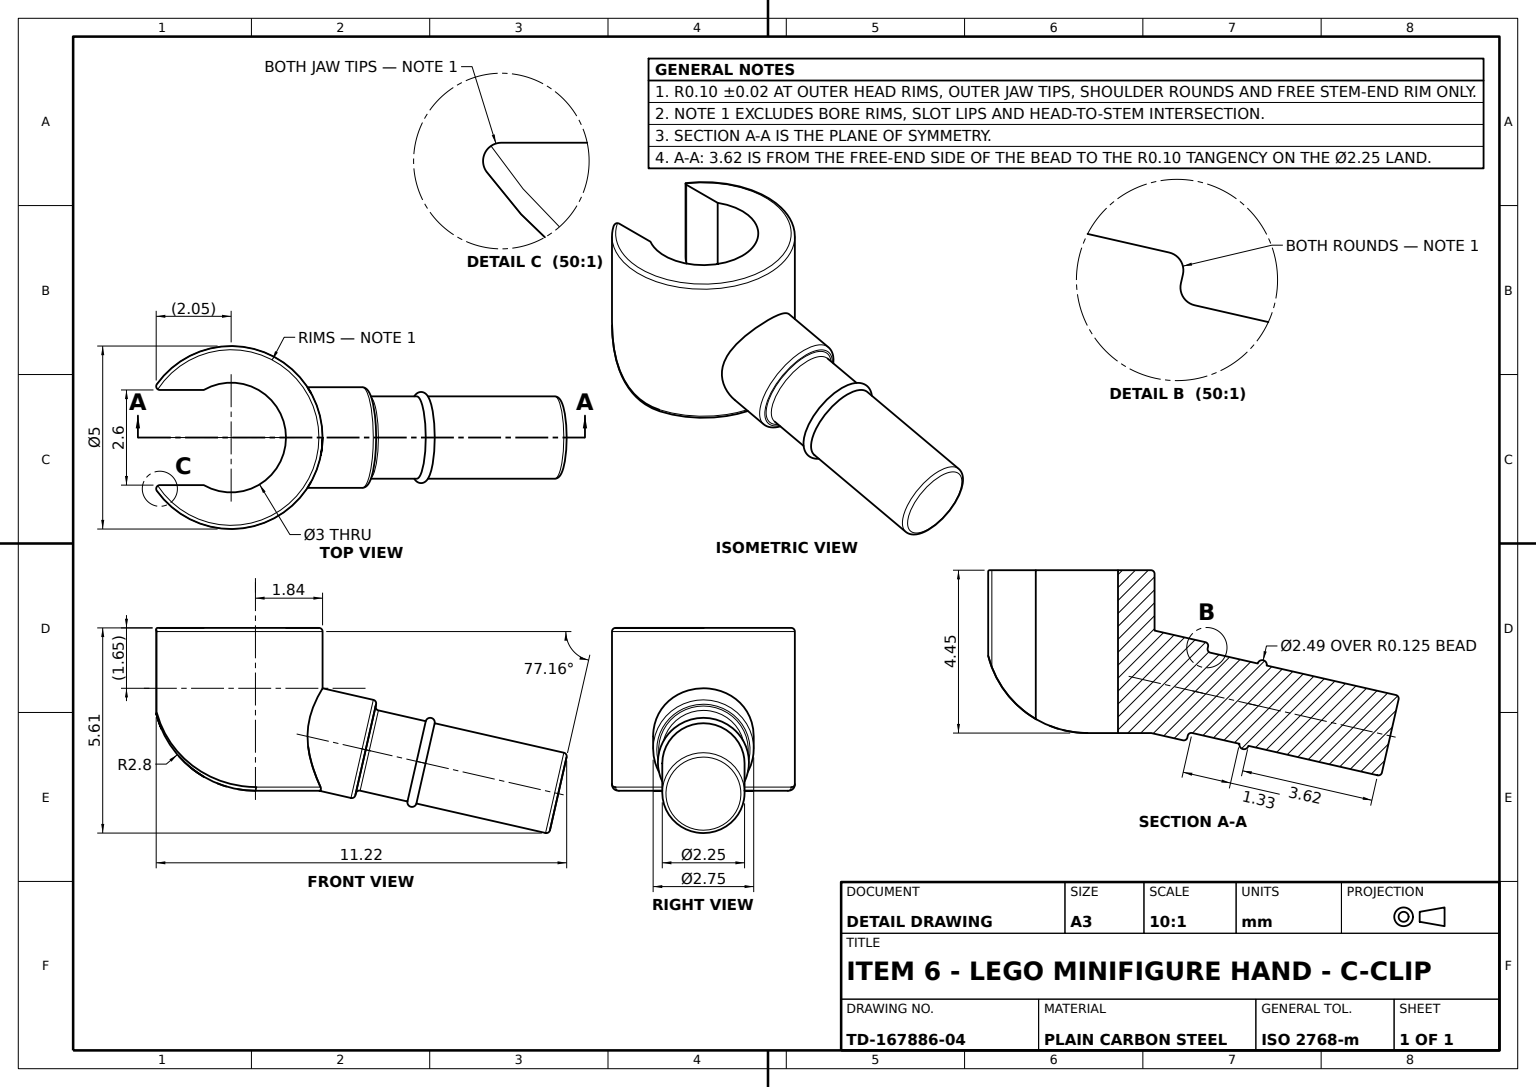
ISO-10303-21;
HEADER;
FILE_DESCRIPTION((''),'2;1');
FILE_NAME('','',(''),(''),'','','');
FILE_SCHEMA(('AUTOMOTIVE_DESIGN'));
ENDSEC;
DATA;
#1=APPLICATION_CONTEXT('');
#2=PRODUCT_CONTEXT('',#1,'mechanical');
#3=PRODUCT('','','',(#2));
#4=PRODUCT_DEFINITION_FORMATION('','',#3);
#5=PRODUCT_DEFINITION_CONTEXT('',#1,'design');
#6=PRODUCT_DEFINITION('','',#4,#5);
#7=PRODUCT_DEFINITION_SHAPE('','',#6);
#8=(LENGTH_UNIT()NAMED_UNIT(*)SI_UNIT(.MILLI.,.METRE.));
#9=(NAMED_UNIT(*)PLANE_ANGLE_UNIT()SI_UNIT($,.RADIAN.));
#10=(NAMED_UNIT(*)SI_UNIT($,.STERADIAN.)SOLID_ANGLE_UNIT());
#11=UNCERTAINTY_MEASURE_WITH_UNIT(LENGTH_MEASURE(1.E-05),#8,'distance_accuracy_value','');
#12=(GEOMETRIC_REPRESENTATION_CONTEXT(3)GLOBAL_UNCERTAINTY_ASSIGNED_CONTEXT((#11))GLOBAL_UNIT_ASSIGNED_CONTEXT((#8,#9,#10))REPRESENTATION_CONTEXT('',''));
#13=CARTESIAN_POINT('',(0.,2.195748,-4.027251));
#14=VERTEX_POINT('',#13);
#15=CARTESIAN_POINT('',(0.,0.002011,-3.527235));
#16=VERTEX_POINT('',#15);
#17=CARTESIAN_POINT('',(0.,1.09888,-3.777243));
#18=DIRECTION('',(0.,-0.222229226,-0.974994447));
#19=DIRECTION('',(0.,0.974994447,-0.222229226));
#20=AXIS2_PLACEMENT_3D('',#17,#18,#19);
#21=CIRCLE('',#20,1.125);
#22=EDGE_CURVE('',#14,#16,#21,.T.);
#23=ORIENTED_EDGE('',*,*,#22,.T.);
#24=CARTESIAN_POINT('',(0.,-0.293063,-4.821825));
#25=VERTEX_POINT('',#24);
#26=CARTESIAN_POINT('',(0.,1.449062,2.821467));
#27=VECTOR('',#18,1000.);
#28=LINE('',#26,#27);
#29=EDGE_CURVE('',#16,#25,#28,.T.);
#30=ORIENTED_EDGE('',*,*,#29,.T.);
#31=CARTESIAN_POINT('',(0.,1.900674,-5.321841));
#32=VERTEX_POINT('',#31);
#33=CARTESIAN_POINT('',(0.,0.803805,-5.071833));
#34=AXIS2_PLACEMENT_3D('',#33,#18,#19);
#35=CIRCLE('',#34,1.125);
#36=EDGE_CURVE('',#32,#25,#35,.T.);
#37=ORIENTED_EDGE('',*,*,#36,.F.);
#38=CARTESIAN_POINT('',(0.,3.6428,2.321451));
#39=LINE('',#38,#27);
#40=EDGE_CURVE('',#14,#32,#39,.T.);
#41=ORIENTED_EDGE('',*,*,#40,.F.);
#42=EDGE_LOOP('',(#23,#30,#37,#41));
#43=FACE_OUTER_BOUND('',#42,.T.);
#44=CARTESIAN_POINT('',(0.,2.545931,2.571459));
#45=AXIS2_PLACEMENT_3D('',#44,#18,#19);
#46=CYLINDRICAL_SURFACE('',#45,1.125);
#47=ADVANCED_FACE('',(#43),#46,.T.);
#48=CARTESIAN_POINT('',(1.3,4.45,1.949359));
#49=VERTEX_POINT('',#48);
#50=CARTESIAN_POINT('',(1.317579,4.45,2.005987));
#51=VERTEX_POINT('',#50);
#52=CARTESIAN_POINT('',(1.4,4.45,1.949359));
#53=DIRECTION('',(0.,1.,0.));
#54=DIRECTION('',(0.,0.,1.));
#55=AXIS2_PLACEMENT_3D('',#52,#53,#54);
#56=CIRCLE('',#55,0.1);
#57=EDGE_CURVE('',#49,#51,#56,.T.);
#58=ORIENTED_EDGE('',*,*,#57,.T.);
#59=CARTESIAN_POINT('',(-1.317579,4.45,2.005987));
#60=VERTEX_POINT('',#59);
#61=CARTESIAN_POINT('',(0.,4.45,0.));
#62=AXIS2_PLACEMENT_3D('',#61,#53,#54);
#63=CIRCLE('',#62,2.4);
#64=EDGE_CURVE('',#51,#60,#63,.T.);
#65=ORIENTED_EDGE('',*,*,#64,.T.);
#66=CARTESIAN_POINT('',(-1.3,4.45,1.949359));
#67=VERTEX_POINT('',#66);
#68=CARTESIAN_POINT('',(-1.4,4.45,1.949359));
#69=AXIS2_PLACEMENT_3D('',#68,#53,#54);
#70=CIRCLE('',#69,0.1);
#71=EDGE_CURVE('',#60,#67,#70,.T.);
#72=ORIENTED_EDGE('',*,*,#71,.T.);
#73=CARTESIAN_POINT('',(-1.3,4.45,0.748331));
#74=VERTEX_POINT('',#73);
#75=DIRECTION('',(0.,0.,-1.));
#76=VECTOR('',#75,1000.);
#77=LINE('',#73,#76);
#78=EDGE_CURVE('',#67,#74,#77,.T.);
#79=ORIENTED_EDGE('',*,*,#78,.T.);
#80=CARTESIAN_POINT('',(0.,4.45,-1.5));
#81=VERTEX_POINT('',#80);
#82=DIRECTION('',(0.,-1.,0.));
#83=AXIS2_PLACEMENT_3D('',#61,#82,#54);
#84=CIRCLE('',#83,1.5);
#85=EDGE_CURVE('',#74,#81,#84,.T.);
#86=ORIENTED_EDGE('',*,*,#85,.T.);
#87=CARTESIAN_POINT('',(1.3,4.45,0.748331));
#88=VERTEX_POINT('',#87);
#89=EDGE_CURVE('',#81,#88,#84,.T.);
#90=ORIENTED_EDGE('',*,*,#89,.T.);
#91=VECTOR('',#54,1000.);
#92=LINE('',#87,#91);
#93=EDGE_CURVE('',#88,#49,#92,.T.);
#94=ORIENTED_EDGE('',*,*,#93,.T.);
#95=EDGE_LOOP('',(#58,#65,#72,#79,#86,#90,#94));
#96=FACE_OUTER_BOUND('',#95,.T.);
#97=PLANE('',#62);
#98=ADVANCED_FACE('',(#96),#97,.T.);
#99=CARTESIAN_POINT('',(0.,2.364221,-3.963086));
#100=VERTEX_POINT('',#99);
#101=CARTESIAN_POINT('',(0.,-0.122015,-3.396401));
#102=VERTEX_POINT('',#101);
#103=CARTESIAN_POINT('',(0.,1.121103,-3.679743));
#104=AXIS2_PLACEMENT_3D('',#103,#18,#19);
#105=CIRCLE('',#104,1.275);
#106=EDGE_CURVE('',#100,#102,#105,.T.);
#107=ORIENTED_EDGE('',*,*,#106,.F.);
#108=CARTESIAN_POINT('',(0.,2.483943,-3.887809));
#109=VERTEX_POINT('',#108);
#110=CARTESIAN_POINT('',(0.,2.386443,-3.865586));
#111=DIRECTION('',(-1.,0.,0.));
#112=AXIS2_PLACEMENT_3D('',#110,#111,#54);
#113=CIRCLE('',#112,0.1);
#114=EDGE_CURVE('',#109,#100,#113,.T.);
#115=ORIENTED_EDGE('',*,*,#114,.F.);
#116=CARTESIAN_POINT('',(0.,-0.197292,-3.276679));
#117=VERTEX_POINT('',#116);
#118=CARTESIAN_POINT('',(0.,1.143326,-3.582244));
#119=DIRECTION('',(0.,0.222229226,0.974994447));
#120=AXIS2_PLACEMENT_3D('',#118,#119,#19);
#121=CIRCLE('',#120,1.375);
#122=EDGE_CURVE('',#117,#109,#121,.T.);
#123=ORIENTED_EDGE('',*,*,#122,.F.);
#124=CARTESIAN_POINT('',(0.,-0.099792,-3.298902));
#125=DIRECTION('',(1.,0.,0.));
#126=AXIS2_PLACEMENT_3D('',#124,#125,#53);
#127=CIRCLE('',#126,0.1);
#128=EDGE_CURVE('',#117,#102,#127,.T.);
#129=ORIENTED_EDGE('',*,*,#128,.T.);
#130=EDGE_LOOP('',(#107,#115,#123,#129));
#131=FACE_OUTER_BOUND('',#130,.T.);
#132=AXIS2_PLACEMENT_3D('',#118,#18,#19);
#133=TOROIDAL_SURFACE('',#132,1.275,0.1);
#134=ADVANCED_FACE('',(#131),#133,.T.);
#135=CARTESIAN_POINT('',(-0.526506,0.1,-2.44393));
#136=VERTEX_POINT('',#135);
#137=CARTESIAN_POINT('',(0.,2.800264,-2.5));
#138=VERTEX_POINT('',#137);
#139=CARTESIAN_POINT('',(-0.671082,0.168564,-2.412783));
#140=CARTESIAN_POINT('',(-0.801192,0.263045,-2.37118));
#141=CARTESIAN_POINT('',(-1.024629,0.486491,-2.283536));
#142=CARTESIAN_POINT('',(-1.117399,0.614003,-2.237964));
#143=CARTESIAN_POINT('',(-1.265176,0.895227,-2.157867));
#144=CARTESIAN_POINT('',(-1.318703,1.046415,-2.124213));
#145=CARTESIAN_POINT('',(-1.363547,1.284275,-2.095484));
#146=CARTESIAN_POINT('',(-1.372576,1.366794,-2.089507));
#147=CARTESIAN_POINT('',(-1.376559,1.530187,-2.086886));
#148=CARTESIAN_POINT('',(-1.371743,1.611454,-2.090103));
#149=CARTESIAN_POINT('',(-1.335246,1.85388,-2.113755));
#150=CARTESIAN_POINT('',(-1.281777,2.007611,-2.148325));
#151=CARTESIAN_POINT('',(-1.122494,2.281938,-2.235678));
#152=CARTESIAN_POINT('',(-1.01807,2.400809,-2.287088));
#153=CARTESIAN_POINT('',(-0.772898,2.595177,-2.381148));
#154=CARTESIAN_POINT('',(-0.630633,2.671441,-2.424087));
#155=CARTESIAN_POINT('',(-0.327188,2.773583,-2.483313));
#156=CARTESIAN_POINT('',(-0.162781,2.800264,-2.5));
#157=B_SPLINE_CURVE_WITH_KNOTS('',3,(#135,#139,#140,#141,#142,#143,#144,#145,#146,#147,#148,#149,#150,#151,#152,#153,#154,#155,#156,#137),.UNSPECIFIED.,.F.,.F.,(4,2,2,2,2,2,2,2,2,4),(0.00032597,0.000812976,0.001299981,0.001786987,0.00203049,0.002273993,0.002760998,0.003248004,0.00373501,0.004222016),.UNSPECIFIED.);
#158=EDGE_CURVE('',#136,#138,#157,.T.);
#159=ORIENTED_EDGE('',*,*,#158,.T.);
#160=CARTESIAN_POINT('',(0.,3.886548,2.265894));
#161=LINE('',#160,#27);
#162=EDGE_CURVE('',#138,#109,#161,.T.);
#163=ORIENTED_EDGE('',*,*,#162,.T.);
#164=EDGE_CURVE('',#109,#117,#121,.T.);
#165=ORIENTED_EDGE('',*,*,#164,.T.);
#166=CARTESIAN_POINT('',(0.,0.000426,-2.409223));
#167=VERTEX_POINT('',#166);
#168=CARTESIAN_POINT('',(0.,1.205314,2.877024));
#169=LINE('',#168,#27);
#170=EDGE_CURVE('',#167,#117,#169,.T.);
#171=ORIENTED_EDGE('',*,*,#170,.F.);
#172=CARTESIAN_POINT('',(-0.045827,0.000426,-2.409223));
#173=CARTESIAN_POINT('',(-0.090693,0.00107,-2.416558));
#174=CARTESIAN_POINT('',(-0.180203,0.006782,-2.431368));
#175=CARTESIAN_POINT('',(-0.224978,0.011871,-2.439042));
#176=CARTESIAN_POINT('',(-0.357289,0.035077,-2.456039));
#177=CARTESIAN_POINT('',(-0.444898,0.061298,-2.461511));
#178=B_SPLINE_CURVE_WITH_KNOTS('',3,(#166,#172,#173,#174,#175,#176,#177,#135),.UNSPECIFIED.,.F.,.F.,(4,2,2,4),(0.,0.000136244,0.000272488,0.000544975),.UNSPECIFIED.);
#179=EDGE_CURVE('',#167,#136,#178,.T.);
#180=ORIENTED_EDGE('',*,*,#179,.T.);
#181=EDGE_LOOP('',(#159,#163,#165,#171,#180));
#182=FACE_OUTER_BOUND('',#181,.T.);
#183=CYLINDRICAL_SURFACE('',#45,1.375);
#184=ADVANCED_FACE('',(#182),#183,.T.);
#185=CARTESIAN_POINT('',(2.306151,0.,-0.66458));
#186=VERTEX_POINT('',#185);
#187=CARTESIAN_POINT('',(2.307419,0.000004,-0.66));
#188=VERTEX_POINT('',#187);
#189=CARTESIAN_POINT('',(2.306574,0.,-0.663053));
#190=CARTESIAN_POINT('',(2.306997,0.,-0.661527));
#191=B_SPLINE_CURVE_WITH_KNOTS('',3,(#185,#189,#190,#187),.UNSPECIFIED.,.F.,.F.,(4,4),(0.,1.),.UNSPECIFIED.);
#192=EDGE_CURVE('',#186,#188,#191,.T.);
#193=ORIENTED_EDGE('',*,*,#192,.F.);
#194=CARTESIAN_POINT('',(2.402241,0.1,-0.692271));
#195=VERTEX_POINT('',#194);
#196=CARTESIAN_POINT('',(2.30615,0.1,-0.664584));
#197=DIRECTION('',(-0.276910146,0.,-0.960895817));
#198=DIRECTION('',(-0.960895817,0.,0.276910146));
#199=AXIS2_PLACEMENT_3D('',#196,#197,#198);
#200=CIRCLE('',#199,0.1);
#201=EDGE_CURVE('',#195,#186,#200,.T.);
#202=ORIENTED_EDGE('',*,*,#201,.F.);
#203=CARTESIAN_POINT('',(1.458333,2.12376,2.030582));
#204=VERTEX_POINT('',#203);
#205=CARTESIAN_POINT('',(1.513587,1.976507,1.9909));
#206=CARTESIAN_POINT('',(1.57929,1.838629,1.9402));
#207=CARTESIAN_POINT('',(1.718161,1.574556,1.818366));
#208=CARTESIAN_POINT('',(1.79159,1.448448,1.746927));
#209=CARTESIAN_POINT('',(1.93489,1.211533,1.586742));
#210=CARTESIAN_POINT('',(2.005369,1.099802,1.497595));
#211=CARTESIAN_POINT('',(2.139139,0.888314,1.299377));
#212=CARTESIAN_POINT('',(2.202968,0.787808,1.189319));
#213=CARTESIAN_POINT('',(2.316314,0.60306,0.949862));
#214=CARTESIAN_POINT('',(2.365377,0.519628,0.821834));
#215=CARTESIAN_POINT('',(2.443611,0.371512,0.546974));
#216=CARTESIAN_POINT('',(2.472557,0.306896,0.399233));
#217=CARTESIAN_POINT('',(2.517721,0.152871,-0.052749));
#218=CARTESIAN_POINT('',(2.492408,0.1,-0.379382));
#219=B_SPLINE_CURVE_WITH_KNOTS('',3,(#203,#205,#206,#207,#208,#209,#210,#211,#212,#213,#214,#215,#216,#217,#218,#194),.UNSPECIFIED.,.F.,.F.,(4,2,2,2,2,2,2,4),(0.,0.000482652,0.000965304,0.001447955,0.001930607,0.002413259,0.002895911,0.003861214),.UNSPECIFIED.);
#220=EDGE_CURVE('',#204,#195,#219,.T.);
#221=ORIENTED_EDGE('',*,*,#220,.F.);
#222=CARTESIAN_POINT('',(1.395828,2.110809,2.049272));
#223=VERTEX_POINT('',#222);
#224=CARTESIAN_POINT('',(1.457496,2.123542,2.031183));
#225=CARTESIAN_POINT('',(1.45665,2.123324,2.031772));
#226=CARTESIAN_POINT('',(1.455794,2.123106,2.032347));
#227=CARTESIAN_POINT('',(1.447312,2.120948,2.038049));
#228=CARTESIAN_POINT('',(1.437839,2.118783,2.042489));
#229=CARTESIAN_POINT('',(1.428001,2.116755,2.045358));
#230=CARTESIAN_POINT('',(1.417658,2.114622,2.048376));
#231=CARTESIAN_POINT('',(1.406657,2.112589,2.049724));
#232=B_SPLINE_CURVE_WITH_KNOTS('',3,(#203,#224,#225,#226,#227,#228,#229,#230,#231,#222),.UNSPECIFIED.,.F.,.F.,(4,3,3,4),(-0.00000316,0.,0.000031339,0.000064338),.UNSPECIFIED.);
#233=EDGE_CURVE('',#204,#223,#232,.T.);
#234=ORIENTED_EDGE('',*,*,#233,.T.);
#235=CARTESIAN_POINT('',(2.351107,0.000263,-0.501648));
#236=CARTESIAN_POINT('',(2.379031,0.013917,-0.34132));
#237=CARTESIAN_POINT('',(2.404689,0.070515,-0.019083));
#238=CARTESIAN_POINT('',(2.402031,0.112332,0.136819));
#239=CARTESIAN_POINT('',(2.371041,0.221622,0.438944));
#240=CARTESIAN_POINT('',(2.342046,0.290173,0.586658));
#241=CARTESIAN_POINT('',(2.264809,0.446445,0.860414));
#242=CARTESIAN_POINT('',(2.216688,0.534285,0.98771));
#243=CARTESIAN_POINT('',(2.106068,0.72838,1.225371));
#244=CARTESIAN_POINT('',(2.044265,0.833356,1.333928));
#245=CARTESIAN_POINT('',(1.915063,1.054127,1.529423));
#246=CARTESIAN_POINT('',(1.847215,1.170575,1.617153));
#247=CARTESIAN_POINT('',(1.709857,1.416934,1.774366));
#248=CARTESIAN_POINT('',(1.639765,1.547861,1.844231));
#249=CARTESIAN_POINT('',(1.508522,1.819961,1.962492));
#250=CARTESIAN_POINT('',(1.447025,1.961337,2.011313));
#251=B_SPLINE_CURVE_WITH_KNOTS('',3,(#187,#235,#236,#237,#238,#239,#240,#241,#242,#243,#244,#245,#246,#247,#248,#249,#250,#222),.UNSPECIFIED.,.F.,.F.,(4,2,2,2,2,2,2,2,4),(0.,0.000489007,0.000978014,0.001467022,0.001956029,0.002445036,0.002934043,0.003423051,0.003912058),.UNSPECIFIED.);
#252=EDGE_CURVE('',#188,#223,#251,.T.);
#253=ORIENTED_EDGE('',*,*,#252,.F.);
#254=EDGE_LOOP('',(#193,#202,#221,#234,#253));
#255=FACE_OUTER_BOUND('',#254,.T.);
#256=CARTESIAN_POINT('',(1.388515,2.132434,2.054672));
#257=CARTESIAN_POINT('',(1.420798,2.142972,2.057259));
#258=CARTESIAN_POINT('',(1.44637,2.156276,2.039121));
#259=CARTESIAN_POINT('',(1.488858,1.831777,1.980862));
#260=CARTESIAN_POINT('',(1.525857,1.842462,1.984738));
#261=CARTESIAN_POINT('',(1.550912,1.866305,1.964968));
#262=CARTESIAN_POINT('',(1.632898,1.555798,1.860944));
#263=CARTESIAN_POINT('',(1.677555,1.566952,1.865212));
#264=CARTESIAN_POINT('',(1.700936,1.600234,1.844528));
#265=CARTESIAN_POINT('',(1.909188,1.058633,1.547648));
#266=CARTESIAN_POINT('',(1.966857,1.071893,1.55893));
#267=CARTESIAN_POINT('',(1.988737,1.120825,1.529833));
#268=CARTESIAN_POINT('',(2.045126,0.834965,1.353865));
#269=CARTESIAN_POINT('',(2.110856,0.847512,1.364677));
#270=CARTESIAN_POINT('',(2.13034,0.905145,1.335185));
#271=CARTESIAN_POINT('',(2.213351,0.540303,0.996031));
#272=CARTESIAN_POINT('',(2.28937,0.553611,1.014535));
#273=CARTESIAN_POINT('',(2.305574,0.621006,0.975753));
#274=CARTESIAN_POINT('',(2.262234,0.451332,0.868073));
#275=CARTESIAN_POINT('',(2.342553,0.463019,0.886004));
#276=CARTESIAN_POINT('',(2.356494,0.535213,0.847224));
#277=CARTESIAN_POINT('',(2.340833,0.292933,0.592353));
#278=CARTESIAN_POINT('',(2.43017,0.299733,0.606691));
#279=CARTESIAN_POINT('',(2.438368,0.382471,0.570273));
#280=CARTESIAN_POINT('',(2.370448,0.223324,0.44317));
#281=CARTESIAN_POINT('',(2.46351,0.228166,0.454886));
#282=CARTESIAN_POINT('',(2.469217,0.315348,0.420424));
#283=CARTESIAN_POINT('',(2.402084,0.112525,0.137823));
#284=CARTESIAN_POINT('',(2.501375,0.112805,0.140264));
#285=CARTESIAN_POINT('',(2.502171,0.208507,0.113714));
#286=CARTESIAN_POINT('',(2.4048,0.070216,-0.019848));
#287=CARTESIAN_POINT('',(2.505758,0.069353,-0.021934));
#288=CARTESIAN_POINT('',(2.505,0.167708,-0.04466));
#289=CARTESIAN_POINT('',(2.378482,0.01326,-0.34601));
#290=CARTESIAN_POINT('',(2.479643,0.011066,-0.361448));
#291=CARTESIAN_POINT('',(2.477585,0.112787,-0.372279));
#292=CARTESIAN_POINT('',(2.349913,0.,-0.507099));
#293=CARTESIAN_POINT('',(2.449692,-0.00157,-0.527614));
#294=CARTESIAN_POINT('',(2.447826,0.1,-0.534087));
#295=CARTESIAN_POINT('',(2.30615,0.,-0.664584));
#296=CARTESIAN_POINT('',(2.40224,0.,-0.692275));
#297=CARTESIAN_POINT('',(2.40224,0.1,-0.692275));
#298=(BOUNDED_SURFACE()B_SPLINE_SURFACE(3,2,((#256,#257,#258),(#259,#260,#261),(#262,#263,#264),(#265,#266,#267),(#268,#269,#270),(#271,#272,#273),(#274,#275,#276),(#277,#278,#279),(#280,#281,#282),(#283,#284,#285),(#286,#287,#288),(#289,#290,#291),(#292,#293,#294),(#295,#296,#297)),.UNSPECIFIED.,.F.,.F.,.T.)B_SPLINE_SURFACE_WITH_KNOTS((4,2,2,2,2,2,4),(3,3),(0.00303462,0.003974751,0.004914882,0.005384947,0.005855013,0.006325078,0.006795144),(0.,1.),.UNSPECIFIED.)GEOMETRIC_REPRESENTATION_ITEM()RATIONAL_B_SPLINE_SURFACE(((1.,0.946606423,1.),(1.,0.933365088,1.),(1.,0.911943949,1.),(1.,0.860602961,1.),(1.,0.830277742,1.),(1.,0.784190406,1.),(1.,0.769139619,1.),(1.,0.741636956,1.),(1.,0.729163986,1.),(1.,0.710585282,1.),(1.,0.704301302,1.),(1.,0.699732621,1.),(1.,0.701577857,1.),(1.,0.707106781,1.)))REPRESENTATION_ITEM('')SURFACE());
#299=ADVANCED_FACE('',(#255),#298,.T.);
#300=CARTESIAN_POINT('',(-1.395828,2.110809,2.049272));
#301=VERTEX_POINT('',#300);
#302=CARTESIAN_POINT('',(-2.307419,0.000004,-0.66));
#303=VERTEX_POINT('',#302);
#304=CARTESIAN_POINT('',(-1.446983,1.961458,2.011344));
#305=CARTESIAN_POINT('',(-1.508479,1.820048,1.962532));
#306=CARTESIAN_POINT('',(-1.639837,1.547715,1.844165));
#307=CARTESIAN_POINT('',(-1.709854,1.416939,1.774374));
#308=CARTESIAN_POINT('',(-1.847278,1.170463,1.617078));
#309=CARTESIAN_POINT('',(-1.915278,1.053756,1.529168));
#310=CARTESIAN_POINT('',(-2.044966,0.83216,1.332795));
#311=CARTESIAN_POINT('',(-2.107174,0.72647,1.223213));
#312=CARTESIAN_POINT('',(-2.217103,0.533527,0.986597));
#313=CARTESIAN_POINT('',(-2.265158,0.445803,0.859475));
#314=CARTESIAN_POINT('',(-2.342496,0.289196,0.584759));
#315=CARTESIAN_POINT('',(-2.371161,0.221268,0.43805));
#316=CARTESIAN_POINT('',(-2.40201,0.112335,0.13674));
#317=CARTESIAN_POINT('',(-2.404635,0.070163,-0.020687));
#318=CARTESIAN_POINT('',(-2.378897,0.013856,-0.342071));
#319=CARTESIAN_POINT('',(-2.351092,0.000263,-0.501702));
#320=B_SPLINE_CURVE_WITH_KNOTS('',3,(#300,#304,#305,#306,#307,#308,#309,#310,#311,#312,#313,#314,#315,#316,#317,#318,#319,#302),.UNSPECIFIED.,.F.,.F.,(4,2,2,2,2,2,2,2,4),(0.000385937,0.000877098,0.00136826,0.001859422,0.002350584,0.002841745,0.003332907,0.003824069,0.00431523),.UNSPECIFIED.);
#321=EDGE_CURVE('',#301,#303,#320,.T.);
#322=ORIENTED_EDGE('',*,*,#321,.T.);
#323=CARTESIAN_POINT('',(-1.346997,0.000004,-0.66));
#324=VERTEX_POINT('',#323);
#325=CARTESIAN_POINT('',(-9.5,0.000004,-0.66));
#326=VECTOR('',#125,1000.);
#327=LINE('',#325,#326);
#328=EDGE_CURVE('',#303,#324,#327,.T.);
#329=ORIENTED_EDGE('',*,*,#328,.T.);
#330=CARTESIAN_POINT('',(-1.3,0.382632,0.748331));
#331=VERTEX_POINT('',#330);
#332=CARTESIAN_POINT('',(-1.357276,0.324476,0.648833));
#333=CARTESIAN_POINT('',(-1.403248,0.270794,0.542979));
#334=CARTESIAN_POINT('',(-1.470904,0.174748,0.316817));
#335=CARTESIAN_POINT('',(-1.492203,0.132406,0.195623));
#336=CARTESIAN_POINT('',(-1.504189,0.065684,-0.048525));
#337=CARTESIAN_POINT('',(-1.495153,0.040279,-0.175015));
#338=CARTESIAN_POINT('',(-1.444479,0.007554,-0.423784));
#339=CARTESIAN_POINT('',(-1.403781,0.000193,-0.544108));
#340=B_SPLINE_CURVE_WITH_KNOTS('',3,(#330,#332,#333,#334,#335,#336,#337,#338,#339,#323),.UNSPECIFIED.,.F.,.F.,(4,2,2,2,4),(0.,0.00038136,0.000762721,0.001144081,0.001525441),.UNSPECIFIED.);
#341=EDGE_CURVE('',#331,#324,#340,.T.);
#342=ORIENTED_EDGE('',*,*,#341,.F.);
#343=CARTESIAN_POINT('',(-1.3,1.796356,1.949359));
#344=VERTEX_POINT('',#343);
#345=CARTESIAN_POINT('',(-1.3,2.8,-0.664584));
#346=AXIS2_PLACEMENT_3D('',#345,#125,#54);
#347=CIRCLE('',#346,2.8);
#348=EDGE_CURVE('',#344,#331,#347,.T.);
#349=ORIENTED_EDGE('',*,*,#348,.F.);
#350=CARTESIAN_POINT('',(-1.3,1.851902,1.970686));
#351=CARTESIAN_POINT('',(-1.306166,1.907372,1.989955));
#352=CARTESIAN_POINT('',(-1.324661,1.990395,2.015972));
#353=CARTESIAN_POINT('',(-1.332363,2.018134,2.02418));
#354=CARTESIAN_POINT('',(-1.348598,2.058151,2.035388));
#355=CARTESIAN_POINT('',(-1.354783,2.071315,2.038964));
#356=CARTESIAN_POINT('',(-1.370709,2.095463,2.045357));
#357=CARTESIAN_POINT('',(-1.38095,2.108362,2.048651));
#358=B_SPLINE_CURVE_WITH_KNOTS('',3,(#343,#350,#351,#352,#353,#354,#355,#356,#357,#300),.UNSPECIFIED.,.F.,.F.,(4,2,2,2,4),(0.,0.000177113,0.000265669,0.000309948,0.000354226),.UNSPECIFIED.);
#359=EDGE_CURVE('',#344,#301,#358,.T.);
#360=ORIENTED_EDGE('',*,*,#359,.T.);
#361=EDGE_LOOP('',(#322,#329,#342,#349,#360));
#362=FACE_OUTER_BOUND('',#361,.T.);
#363=CARTESIAN_POINT('',(-9.5,2.8,-0.664584));
#364=AXIS2_PLACEMENT_3D('',#363,#125,#75);
#365=CYLINDRICAL_SURFACE('',#364,2.8);
#366=ADVANCED_FACE('',(#362),#365,.T.);
#367=ORIENTED_EDGE('',*,*,#29,.F.);
#368=EDGE_CURVE('',#16,#14,#21,.T.);
#369=ORIENTED_EDGE('',*,*,#368,.T.);
#370=ORIENTED_EDGE('',*,*,#40,.T.);
#371=EDGE_CURVE('',#25,#32,#35,.T.);
#372=ORIENTED_EDGE('',*,*,#371,.F.);
#373=EDGE_LOOP('',(#367,#369,#370,#372));
#374=FACE_OUTER_BOUND('',#373,.T.);
#375=ADVANCED_FACE('',(#374),#46,.T.);
#376=CARTESIAN_POINT('',(0.,4.35,-2.5));
#377=VERTEX_POINT('',#376);
#378=CARTESIAN_POINT('',(1.458333,4.35,2.030582));
#379=VERTEX_POINT('',#378);
#380=CARTESIAN_POINT('',(0.,4.35,0.));
#381=AXIS2_PLACEMENT_3D('',#380,#82,#54);
#382=CIRCLE('',#381,2.5);
#383=EDGE_CURVE('',#377,#379,#382,.T.);
#384=ORIENTED_EDGE('',*,*,#383,.T.);
#385=CARTESIAN_POINT('',(1.458333,4.45,2.030582));
#386=VECTOR('',#82,1000.);
#387=LINE('',#385,#386);
#388=EDGE_CURVE('',#379,#204,#387,.T.);
#389=ORIENTED_EDGE('',*,*,#388,.T.);
#390=ORIENTED_EDGE('',*,*,#220,.T.);
#391=CARTESIAN_POINT('',(0.526506,0.1,-2.44393));
#392=VERTEX_POINT('',#391);
#393=CARTESIAN_POINT('',(0.,0.1,0.));
#394=AXIS2_PLACEMENT_3D('',#393,#53,#54);
#395=CIRCLE('',#394,2.5);
#396=EDGE_CURVE('',#195,#392,#395,.T.);
#397=ORIENTED_EDGE('',*,*,#396,.T.);
#398=CARTESIAN_POINT('',(0.162618,2.800264,-2.5));
#399=CARTESIAN_POINT('',(0.327027,2.773614,-2.483333));
#400=CARTESIAN_POINT('',(0.630419,2.671536,-2.424141));
#401=CARTESIAN_POINT('',(0.772795,2.595166,-2.381159));
#402=CARTESIAN_POINT('',(1.017217,2.401579,-2.287444));
#403=CARTESIAN_POINT('',(1.122044,2.282116,-2.235869));
#404=CARTESIAN_POINT('',(1.279864,2.011493,-2.149428));
#405=CARTESIAN_POINT('',(1.334241,1.856863,-2.114394));
#406=CARTESIAN_POINT('',(1.371223,1.616676,-2.090446));
#407=CARTESIAN_POINT('',(1.376446,1.533581,-2.08696));
#408=CARTESIAN_POINT('',(1.372848,1.370241,-2.089329));
#409=CARTESIAN_POINT('',(1.36427,1.289294,-2.095014));
#410=CARTESIAN_POINT('',(1.319514,1.048435,-2.123709));
#411=CARTESIAN_POINT('',(1.265531,0.895975,-2.157668));
#412=CARTESIAN_POINT('',(1.117365,0.613866,-2.237989));
#413=CARTESIAN_POINT('',(1.025116,0.486983,-2.283344));
#414=CARTESIAN_POINT('',(0.800751,0.262599,-2.371354));
#415=CARTESIAN_POINT('',(0.672596,0.169282,-2.412457));
#416=B_SPLINE_CURVE_WITH_KNOTS('',3,(#137,#398,#399,#400,#401,#402,#403,#404,#405,#406,#407,#408,#409,#410,#411,#412,#413,#414,#415,#391),.UNSPECIFIED.,.F.,.F.,(4,2,2,2,2,2,2,2,2,4),(0.004222016,0.004708533,0.00519505,0.005681568,0.006168085,0.006411344,0.006654603,0.00714112,0.007627637,0.008114155),.UNSPECIFIED.);
#417=EDGE_CURVE('',#138,#392,#416,.T.);
#418=ORIENTED_EDGE('',*,*,#417,.F.);
#419=CARTESIAN_POINT('',(0.,4.45,-2.5));
#420=LINE('',#419,#386);
#421=EDGE_CURVE('',#377,#138,#420,.T.);
#422=ORIENTED_EDGE('',*,*,#421,.F.);
#423=EDGE_LOOP('',(#384,#389,#390,#397,#418,#422));
#424=FACE_OUTER_BOUND('',#423,.T.);
#425=AXIS2_PLACEMENT_3D('',#61,#82,#75);
#426=CYLINDRICAL_SURFACE('',#425,2.5);
#427=ADVANCED_FACE('',(#424),#426,.T.);
#428=CARTESIAN_POINT('',(0.,1.845161,-5.565395));
#429=VERTEX_POINT('',#428);
#430=CARTESIAN_POINT('',(0.,1.040156,-9.097222));
#431=VERTEX_POINT('',#430);
#432=EDGE_CURVE('',#429,#431,#39,.T.);
#433=ORIENTED_EDGE('',*,*,#432,.T.);
#434=CARTESIAN_POINT('',(0.,-1.153581,-8.597206));
#435=VERTEX_POINT('',#434);
#436=CARTESIAN_POINT('',(0.,-0.056712,-8.847214));
#437=AXIS2_PLACEMENT_3D('',#436,#119,#19);
#438=CIRCLE('',#437,1.125);
#439=EDGE_CURVE('',#431,#435,#438,.T.);
#440=ORIENTED_EDGE('',*,*,#439,.T.);
#441=CARTESIAN_POINT('',(0.,-0.348576,-5.065379));
#442=VERTEX_POINT('',#441);
#443=EDGE_CURVE('',#442,#435,#28,.T.);
#444=ORIENTED_EDGE('',*,*,#443,.F.);
#445=CARTESIAN_POINT('',(0.,0.748293,-5.315387));
#446=DIRECTION('',(0.,-0.974994447,0.222229226));
#447=AXIS2_PLACEMENT_3D('',#445,#119,#446);
#448=CIRCLE('',#447,1.125);
#449=EDGE_CURVE('',#429,#442,#448,.T.);
#450=ORIENTED_EDGE('',*,*,#449,.F.);
#451=EDGE_LOOP('',(#433,#440,#444,#450));
#452=FACE_OUTER_BOUND('',#451,.T.);
#453=ADVANCED_FACE('',(#452),#46,.T.);
#454=CARTESIAN_POINT('',(1.3,0.382632,0.748331));
#455=VERTEX_POINT('',#454);
#456=CARTESIAN_POINT('',(1.3,1.796356,1.949359));
#457=VERTEX_POINT('',#456);
#458=CARTESIAN_POINT('',(1.3,2.8,-0.664584));
#459=AXIS2_PLACEMENT_3D('',#458,#111,#75);
#460=CIRCLE('',#459,2.8);
#461=EDGE_CURVE('',#455,#457,#460,.T.);
#462=ORIENTED_EDGE('',*,*,#461,.T.);
#463=VECTOR('',#53,1000.);
#464=LINE('',#48,#463);
#465=EDGE_CURVE('',#457,#49,#464,.T.);
#466=ORIENTED_EDGE('',*,*,#465,.T.);
#467=ORIENTED_EDGE('',*,*,#93,.F.);
#468=LINE('',#87,#386);
#469=EDGE_CURVE('',#88,#455,#468,.T.);
#470=ORIENTED_EDGE('',*,*,#469,.T.);
#471=EDGE_LOOP('',(#462,#466,#467,#470));
#472=FACE_OUTER_BOUND('',#471,.T.);
#473=AXIS2_PLACEMENT_3D('',#87,#125,#75);
#474=PLANE('',#473);
#475=ADVANCED_FACE('',(#472),#474,.F.);
#476=CARTESIAN_POINT('',(0.445012,0.061353,-2.461486));
#477=CARTESIAN_POINT('',(0.35629,0.034808,-2.455971));
#478=CARTESIAN_POINT('',(0.223754,0.011704,-2.438854));
#479=CARTESIAN_POINT('',(0.179508,0.006723,-2.431249));
#480=CARTESIAN_POINT('',(0.090483,0.001071,-2.416527));
#481=CARTESIAN_POINT('',(0.045723,0.000426,-2.409223));
#482=B_SPLINE_CURVE_WITH_KNOTS('',3,(#391,#476,#477,#478,#479,#480,#481,#166),.UNSPECIFIED.,.F.,.F.,(4,2,2,4),(-0.000543733,-0.000271866,-0.000135933,0.),.UNSPECIFIED.);
#483=EDGE_CURVE('',#392,#167,#482,.T.);
#484=ORIENTED_EDGE('',*,*,#483,.F.);
#485=ORIENTED_EDGE('',*,*,#396,.F.);
#486=ORIENTED_EDGE('',*,*,#201,.T.);
#487=CARTESIAN_POINT('',(-2.306151,0.,-0.66458));
#488=VERTEX_POINT('',#487);
#489=CARTESIAN_POINT('',(0.,0.,0.));
#490=AXIS2_PLACEMENT_3D('',#489,#82,#54);
#491=CIRCLE('',#490,2.4);
#492=EDGE_CURVE('',#488,#186,#491,.T.);
#493=ORIENTED_EDGE('',*,*,#492,.F.);
#494=CARTESIAN_POINT('',(-2.402241,0.1,-0.692271));
#495=VERTEX_POINT('',#494);
#496=CARTESIAN_POINT('',(-2.30615,0.1,-0.664584));
#497=DIRECTION('',(0.276910146,0.,-0.960895817));
#498=DIRECTION('',(0.960895817,0.,0.276910146));
#499=AXIS2_PLACEMENT_3D('',#496,#497,#498);
#500=CIRCLE('',#499,0.1);
#501=EDGE_CURVE('',#488,#495,#500,.T.);
#502=ORIENTED_EDGE('',*,*,#501,.T.);
#503=EDGE_CURVE('',#136,#495,#395,.T.);
#504=ORIENTED_EDGE('',*,*,#503,.F.);
#505=ORIENTED_EDGE('',*,*,#179,.F.);
#506=EDGE_LOOP('',(#484,#485,#486,#493,#502,#504,#505));
#507=FACE_OUTER_BOUND('',#506,.T.);
#508=TOROIDAL_SURFACE('',#394,2.4,0.1);
#509=ADVANCED_FACE('',(#507),#508,.T.);
#510=CARTESIAN_POINT('',(0.,1.868043,-5.442507));
#511=AXIS2_PLACEMENT_3D('',#510,#125,#53);
#512=CIRCLE('',#511,0.125);
#513=EDGE_CURVE('',#429,#32,#512,.T.);
#514=ORIENTED_EDGE('',*,*,#513,.T.);
#515=ORIENTED_EDGE('',*,*,#36,.T.);
#516=CARTESIAN_POINT('',(0.,-0.315945,-4.944713));
#517=AXIS2_PLACEMENT_3D('',#516,#111,#54);
#518=CIRCLE('',#517,0.125);
#519=EDGE_CURVE('',#442,#25,#518,.T.);
#520=ORIENTED_EDGE('',*,*,#519,.F.);
#521=EDGE_CURVE('',#442,#429,#448,.T.);
#522=ORIENTED_EDGE('',*,*,#521,.T.);
#523=EDGE_LOOP('',(#514,#515,#520,#522));
#524=FACE_OUTER_BOUND('',#523,.T.);
#525=CARTESIAN_POINT('',(0.,0.776049,-5.19361));
#526=AXIS2_PLACEMENT_3D('',#525,#119,#446);
#527=TOROIDAL_SURFACE('',#526,1.12,0.125);
#528=ADVANCED_FACE('',(#524),#527,.T.);
#529=CARTESIAN_POINT('',(0.,0.,-1.5));
#530=VERTEX_POINT('',#529);
#531=LINE('',#80,#386);
#532=EDGE_CURVE('',#81,#530,#531,.T.);
#533=ORIENTED_EDGE('',*,*,#532,.T.);
#534=CARTESIAN_POINT('',(1.346997,0.,-0.66));
#535=VERTEX_POINT('',#534);
#536=CIRCLE('',#490,1.5);
#537=EDGE_CURVE('',#530,#535,#536,.T.);
#538=ORIENTED_EDGE('',*,*,#537,.T.);
#539=CARTESIAN_POINT('',(1.403626,0.000193,-0.544424));
#540=CARTESIAN_POINT('',(1.444271,0.007514,-0.424409));
#541=CARTESIAN_POINT('',(1.494987,0.040078,-0.176228));
#542=CARTESIAN_POINT('',(1.504177,0.065331,-0.049998));
#543=CARTESIAN_POINT('',(1.492313,0.132203,0.195062));
#544=CARTESIAN_POINT('',(1.47107,0.17444,0.315961));
#545=CARTESIAN_POINT('',(1.40371,0.270211,0.541734));
#546=CARTESIAN_POINT('',(1.357179,0.324574,0.649));
#547=B_SPLINE_CURVE_WITH_KNOTS('',3,(#534,#539,#540,#541,#542,#543,#544,#545,#546,#454),.UNSPECIFIED.,.F.,.F.,(4,2,2,2,4),(0.,0.000380604,0.000761208,0.001141813,0.001522417),.UNSPECIFIED.);
#548=EDGE_CURVE('',#535,#455,#547,.T.);
#549=ORIENTED_EDGE('',*,*,#548,.T.);
#550=ORIENTED_EDGE('',*,*,#469,.F.);
#551=ORIENTED_EDGE('',*,*,#89,.F.);
#552=EDGE_LOOP('',(#533,#538,#549,#550,#551));
#553=FACE_OUTER_BOUND('',#552,.T.);
#554=CYLINDRICAL_SURFACE('',#425,1.5);
#555=ADVANCED_FACE('',(#553),#554,.F.);
#556=ORIENTED_EDGE('',*,*,#548,.F.);
#557=EDGE_CURVE('',#535,#188,#327,.T.);
#558=ORIENTED_EDGE('',*,*,#557,.T.);
#559=ORIENTED_EDGE('',*,*,#252,.T.);
#560=CARTESIAN_POINT('',(1.380794,2.108337,2.048644));
#561=CARTESIAN_POINT('',(1.370597,2.095332,2.045323));
#562=CARTESIAN_POINT('',(1.354664,2.071092,2.038904));
#563=CARTESIAN_POINT('',(1.348455,2.057833,2.035301));
#564=CARTESIAN_POINT('',(1.33231,2.017936,2.024121));
#565=CARTESIAN_POINT('',(1.324716,1.990591,2.01603));
#566=CARTESIAN_POINT('',(1.306236,1.907786,1.990091));
#567=CARTESIAN_POINT('',(1.3,1.851816,1.970653));
#568=B_SPLINE_CURVE_WITH_KNOTS('',3,(#222,#560,#561,#562,#563,#564,#565,#566,#567,#456),.UNSPECIFIED.,.F.,.F.,(4,2,2,2,4),(0.,0.000044959,0.000089918,0.000179837,0.000359673),.UNSPECIFIED.);
#569=EDGE_CURVE('',#223,#457,#568,.T.);
#570=ORIENTED_EDGE('',*,*,#569,.T.);
#571=ORIENTED_EDGE('',*,*,#461,.F.);
#572=EDGE_LOOP('',(#556,#558,#559,#570,#571));
#573=FACE_OUTER_BOUND('',#572,.T.);
#574=ADVANCED_FACE('',(#573),#365,.T.);
#575=EDGE_CURVE('',#324,#530,#536,.T.);
#576=ORIENTED_EDGE('',*,*,#575,.F.);
#577=ORIENTED_EDGE('',*,*,#328,.F.);
#578=CARTESIAN_POINT('',(-2.306997,0.,-0.661527));
#579=CARTESIAN_POINT('',(-2.306574,0.,-0.663053));
#580=B_SPLINE_CURVE_WITH_KNOTS('',3,(#302,#578,#579,#487),.UNSPECIFIED.,.F.,.F.,(4,4),(0.,1.),.UNSPECIFIED.);
#581=EDGE_CURVE('',#303,#488,#580,.T.);
#582=ORIENTED_EDGE('',*,*,#581,.T.);
#583=ORIENTED_EDGE('',*,*,#492,.T.);
#584=ORIENTED_EDGE('',*,*,#192,.T.);
#585=ORIENTED_EDGE('',*,*,#557,.F.);
#586=ORIENTED_EDGE('',*,*,#537,.F.);
#587=EDGE_LOOP('',(#576,#577,#582,#583,#584,#585,#586));
#588=FACE_OUTER_BOUND('',#587,.T.);
#589=AXIS2_PLACEMENT_3D('',#489,#53,#54);
#590=PLANE('',#589);
#591=ADVANCED_FACE('',(#588),#590,.F.);
#592=ORIENTED_EDGE('',*,*,#164,.F.);
#593=ORIENTED_EDGE('',*,*,#114,.T.);
#594=EDGE_CURVE('',#102,#100,#105,.T.);
#595=ORIENTED_EDGE('',*,*,#594,.F.);
#596=ORIENTED_EDGE('',*,*,#128,.F.);
#597=EDGE_LOOP('',(#592,#593,#595,#596));
#598=FACE_OUTER_BOUND('',#597,.T.);
#599=ADVANCED_FACE('',(#598),#133,.T.);
#600=ORIENTED_EDGE('',*,*,#465,.F.);
#601=ORIENTED_EDGE('',*,*,#569,.F.);
#602=ORIENTED_EDGE('',*,*,#233,.F.);
#603=ORIENTED_EDGE('',*,*,#388,.F.);
#604=CARTESIAN_POINT('',(1.322629,4.45,2.013337));
#605=CARTESIAN_POINT('',(1.328781,4.448752,2.020085));
#606=CARTESIAN_POINT('',(1.335365,4.446503,2.025663));
#607=CARTESIAN_POINT('',(1.341918,4.444265,2.031213));
#608=CARTESIAN_POINT('',(1.349058,4.441003,2.03578));
#609=CARTESIAN_POINT('',(1.356236,4.437125,2.039274));
#610=CARTESIAN_POINT('',(1.366351,4.43166,2.044197));
#611=CARTESIAN_POINT('',(1.37682,4.424838,2.04716));
#612=CARTESIAN_POINT('',(1.386849,4.417485,2.04849));
#613=CARTESIAN_POINT('',(1.400592,4.407409,2.050314));
#614=CARTESIAN_POINT('',(1.413964,4.396026,2.049178));
#615=CARTESIAN_POINT('',(1.426132,4.384415,2.045884));
#616=CARTESIAN_POINT('',(1.43738,4.373682,2.042839));
#617=CARTESIAN_POINT('',(1.447856,4.362515,2.037891));
#618=CARTESIAN_POINT('',(1.457143,4.351429,2.031424));
#619=CARTESIAN_POINT('',(1.457542,4.350952,2.031146));
#620=CARTESIAN_POINT('',(1.457939,4.350476,2.030866));
#621=B_SPLINE_CURVE_WITH_KNOTS('',3,(#50,#604,#605,#606,#607,#608,#609,#610,#611,#612,#613,#614,#615,#616,#617,#618,#619,#620,#378),.UNSPECIFIED.,.F.,.F.,(4,3,3,3,3,3,4),(0.,0.000026752,0.000053279,0.000090812,0.000142387,0.000189868,0.00019191),.UNSPECIFIED.);
#622=EDGE_CURVE('',#51,#379,#621,.T.);
#623=ORIENTED_EDGE('',*,*,#622,.F.);
#624=ORIENTED_EDGE('',*,*,#57,.F.);
#625=EDGE_LOOP('',(#600,#601,#602,#603,#623,#624));
#626=FACE_OUTER_BOUND('',#625,.T.);
#627=AXIS2_PLACEMENT_3D('',#52,#82,#75);
#628=CYLINDRICAL_SURFACE('',#627,0.1);
#629=ADVANCED_FACE('',(#626),#628,.T.);
#630=CARTESIAN_POINT('',(0.,-0.073266,-3.407512));
#631=VERTEX_POINT('',#630);
#632=CARTESIAN_POINT('',(0.,-0.095488,-3.505012));
#633=AXIS2_PLACEMENT_3D('',#632,#125,#53);
#634=CIRCLE('',#633,0.1);
#635=EDGE_CURVE('',#16,#631,#634,.T.);
#636=ORIENTED_EDGE('',*,*,#635,.F.);
#637=ORIENTED_EDGE('',*,*,#22,.F.);
#638=CARTESIAN_POINT('',(0.,2.315471,-3.951974));
#639=VERTEX_POINT('',#638);
#640=CARTESIAN_POINT('',(0.,2.293248,-4.049474));
#641=AXIS2_PLACEMENT_3D('',#640,#111,#54);
#642=CIRCLE('',#641,0.1);
#643=EDGE_CURVE('',#14,#639,#642,.T.);
#644=ORIENTED_EDGE('',*,*,#643,.T.);
#645=AXIS2_PLACEMENT_3D('',#103,#119,#19);
#646=CIRCLE('',#645,1.225);
#647=EDGE_CURVE('',#631,#639,#646,.T.);
#648=ORIENTED_EDGE('',*,*,#647,.F.);
#649=EDGE_LOOP('',(#636,#637,#644,#648));
#650=FACE_OUTER_BOUND('',#649,.T.);
#651=TOROIDAL_SURFACE('',#20,1.225,0.1);
#652=ADVANCED_FACE('',(#650),#651,.F.);
#653=ORIENTED_EDGE('',*,*,#85,.F.);
#654=LINE('',#73,#386);
#655=EDGE_CURVE('',#74,#331,#654,.T.);
#656=ORIENTED_EDGE('',*,*,#655,.T.);
#657=ORIENTED_EDGE('',*,*,#341,.T.);
#658=ORIENTED_EDGE('',*,*,#575,.T.);
#659=ORIENTED_EDGE('',*,*,#532,.F.);
#660=EDGE_LOOP('',(#653,#656,#657,#658,#659));
#661=FACE_OUTER_BOUND('',#660,.T.);
#662=ADVANCED_FACE('',(#661),#554,.F.);
#663=ORIENTED_EDGE('',*,*,#71,.F.);
#664=CARTESIAN_POINT('',(-1.458333,4.35,2.030582));
#665=VERTEX_POINT('',#664);
#666=CARTESIAN_POINT('',(-1.322629,4.45,2.013337));
#667=CARTESIAN_POINT('',(-1.328781,4.448752,2.020085));
#668=CARTESIAN_POINT('',(-1.335365,4.446503,2.025663));
#669=CARTESIAN_POINT('',(-1.341918,4.444265,2.031213));
#670=CARTESIAN_POINT('',(-1.349058,4.441003,2.03578));
#671=CARTESIAN_POINT('',(-1.356236,4.437125,2.039274));
#672=CARTESIAN_POINT('',(-1.366351,4.43166,2.044197));
#673=CARTESIAN_POINT('',(-1.37682,4.424838,2.04716));
#674=CARTESIAN_POINT('',(-1.386849,4.417485,2.04849));
#675=CARTESIAN_POINT('',(-1.400592,4.407409,2.050314));
#676=CARTESIAN_POINT('',(-1.413964,4.396026,2.049178));
#677=CARTESIAN_POINT('',(-1.426132,4.384415,2.045884));
#678=CARTESIAN_POINT('',(-1.43738,4.373682,2.042839));
#679=CARTESIAN_POINT('',(-1.447856,4.362515,2.037891));
#680=CARTESIAN_POINT('',(-1.457143,4.351429,2.031424));
#681=CARTESIAN_POINT('',(-1.457542,4.350952,2.031146));
#682=CARTESIAN_POINT('',(-1.457939,4.350476,2.030866));
#683=B_SPLINE_CURVE_WITH_KNOTS('',3,(#59,#666,#667,#668,#669,#670,#671,#672,#673,#674,#675,#676,#677,#678,#679,#680,#681,#682,#664),.UNSPECIFIED.,.F.,.F.,(4,3,3,3,3,3,4),(0.,0.000026752,0.000053279,0.000090812,0.000142387,0.000189868,0.00019191),.UNSPECIFIED.);
#684=EDGE_CURVE('',#60,#665,#683,.T.);
#685=ORIENTED_EDGE('',*,*,#684,.T.);
#686=CARTESIAN_POINT('',(-1.458333,2.12376,2.030582));
#687=VERTEX_POINT('',#686);
#688=CARTESIAN_POINT('',(-1.458333,4.45,2.030582));
#689=LINE('',#688,#463);
#690=EDGE_CURVE('',#687,#665,#689,.T.);
#691=ORIENTED_EDGE('',*,*,#690,.F.);
#692=CARTESIAN_POINT('',(-1.407219,2.112682,2.049747));
#693=CARTESIAN_POINT('',(-1.418807,2.114836,2.048226));
#694=CARTESIAN_POINT('',(-1.429629,2.117092,2.044869));
#695=CARTESIAN_POINT('',(-1.438879,2.119021,2.041999));
#696=CARTESIAN_POINT('',(-1.447776,2.121066,2.037737));
#697=CARTESIAN_POINT('',(-1.455794,2.123106,2.032347));
#698=CARTESIAN_POINT('',(-1.45665,2.123324,2.031772));
#699=CARTESIAN_POINT('',(-1.457496,2.123542,2.031183));
#700=B_SPLINE_CURVE_WITH_KNOTS('',3,(#300,#692,#693,#694,#695,#696,#697,#698,#699,#686),.UNSPECIFIED.,.F.,.F.,(4,3,3,4),(0.,0.000034661,0.000064165,0.000067325),.UNSPECIFIED.);
#701=EDGE_CURVE('',#301,#687,#700,.T.);
#702=ORIENTED_EDGE('',*,*,#701,.F.);
#703=ORIENTED_EDGE('',*,*,#359,.F.);
#704=LINE('',#66,#386);
#705=EDGE_CURVE('',#67,#344,#704,.T.);
#706=ORIENTED_EDGE('',*,*,#705,.F.);
#707=EDGE_LOOP('',(#663,#685,#691,#702,#703,#706));
#708=FACE_OUTER_BOUND('',#707,.T.);
#709=AXIS2_PLACEMENT_3D('',#68,#82,#75);
#710=CYLINDRICAL_SURFACE('',#709,0.1);
#711=ADVANCED_FACE('',(#708),#710,.T.);
#712=ORIENTED_EDGE('',*,*,#64,.F.);
#713=ORIENTED_EDGE('',*,*,#622,.T.);
#714=ORIENTED_EDGE('',*,*,#383,.F.);
#715=EDGE_CURVE('',#665,#377,#382,.T.);
#716=ORIENTED_EDGE('',*,*,#715,.F.);
#717=ORIENTED_EDGE('',*,*,#684,.F.);
#718=EDGE_LOOP('',(#712,#713,#714,#716,#717));
#719=FACE_OUTER_BOUND('',#718,.T.);
#720=AXIS2_PLACEMENT_3D('',#380,#53,#54);
#721=TOROIDAL_SURFACE('',#720,2.4,0.1);
#722=ADVANCED_FACE('',(#719),#721,.T.);
#723=ORIENTED_EDGE('',*,*,#647,.T.);
#724=EDGE_CURVE('',#639,#631,#646,.T.);
#725=ORIENTED_EDGE('',*,*,#724,.T.);
#726=EDGE_LOOP('',(#723,#725));
#727=FACE_BOUND('',#726,.T.);
#728=ORIENTED_EDGE('',*,*,#594,.T.);
#729=ORIENTED_EDGE('',*,*,#106,.T.);
#730=EDGE_LOOP('',(#728,#729));
#731=FACE_OUTER_BOUND('',#730,.T.);
#732=PLANE('',#104);
#733=ADVANCED_FACE('',(#727,#731),#732,.T.);
#734=ORIENTED_EDGE('',*,*,#513,.F.);
#735=ORIENTED_EDGE('',*,*,#449,.T.);
#736=ORIENTED_EDGE('',*,*,#519,.T.);
#737=ORIENTED_EDGE('',*,*,#371,.T.);
#738=EDGE_LOOP('',(#734,#735,#736,#737));
#739=FACE_OUTER_BOUND('',#738,.T.);
#740=ADVANCED_FACE('',(#739),#527,.T.);
#741=CARTESIAN_POINT('',(0.,-1.078304,-8.716928));
#742=VERTEX_POINT('',#741);
#743=CARTESIAN_POINT('',(0.,0.920434,-9.172498));
#744=VERTEX_POINT('',#743);
#745=CARTESIAN_POINT('',(0.,-0.078935,-8.944713));
#746=AXIS2_PLACEMENT_3D('',#745,#18,#19);
#747=CIRCLE('',#746,1.025);
#748=EDGE_CURVE('',#742,#744,#747,.T.);
#749=ORIENTED_EDGE('',*,*,#748,.F.);
#750=CARTESIAN_POINT('',(0.,-1.056082,-8.619429));
#751=AXIS2_PLACEMENT_3D('',#750,#125,#53);
#752=CIRCLE('',#751,0.1);
#753=EDGE_CURVE('',#435,#742,#752,.T.);
#754=ORIENTED_EDGE('',*,*,#753,.F.);
#755=ORIENTED_EDGE('',*,*,#439,.F.);
#756=CARTESIAN_POINT('',(0.,0.942657,-9.074999));
#757=AXIS2_PLACEMENT_3D('',#756,#111,#54);
#758=CIRCLE('',#757,0.1);
#759=EDGE_CURVE('',#431,#744,#758,.T.);
#760=ORIENTED_EDGE('',*,*,#759,.T.);
#761=EDGE_LOOP('',(#749,#754,#755,#760));
#762=FACE_OUTER_BOUND('',#761,.T.);
#763=AXIS2_PLACEMENT_3D('',#436,#18,#19);
#764=TOROIDAL_SURFACE('',#763,1.025,0.1);
#765=ADVANCED_FACE('',(#762),#764,.T.);
#766=ORIENTED_EDGE('',*,*,#368,.F.);
#767=ORIENTED_EDGE('',*,*,#635,.T.);
#768=ORIENTED_EDGE('',*,*,#724,.F.);
#769=ORIENTED_EDGE('',*,*,#643,.F.);
#770=EDGE_LOOP('',(#766,#767,#768,#769));
#771=FACE_OUTER_BOUND('',#770,.T.);
#772=ADVANCED_FACE('',(#771),#651,.F.);
#773=ORIENTED_EDGE('',*,*,#759,.F.);
#774=EDGE_CURVE('',#435,#431,#438,.T.);
#775=ORIENTED_EDGE('',*,*,#774,.F.);
#776=ORIENTED_EDGE('',*,*,#753,.T.);
#777=EDGE_CURVE('',#744,#742,#747,.T.);
#778=ORIENTED_EDGE('',*,*,#777,.F.);
#779=EDGE_LOOP('',(#773,#775,#776,#778));
#780=FACE_OUTER_BOUND('',#779,.T.);
#781=ADVANCED_FACE('',(#780),#764,.T.);
#782=ORIENTED_EDGE('',*,*,#521,.F.);
#783=ORIENTED_EDGE('',*,*,#443,.T.);
#784=ORIENTED_EDGE('',*,*,#774,.T.);
#785=ORIENTED_EDGE('',*,*,#432,.F.);
#786=EDGE_LOOP('',(#782,#783,#784,#785));
#787=FACE_OUTER_BOUND('',#786,.T.);
#788=ADVANCED_FACE('',(#787),#46,.T.);
#789=ORIENTED_EDGE('',*,*,#748,.T.);
#790=ORIENTED_EDGE('',*,*,#777,.T.);
#791=EDGE_LOOP('',(#789,#790));
#792=FACE_OUTER_BOUND('',#791,.T.);
#793=CARTESIAN_POINT('',(0.,-1.94197,-8.520074));
#794=AXIS2_PLACEMENT_3D('',#793,#18,#19);
#795=PLANE('',#794);
#796=ADVANCED_FACE('',(#792),#795,.T.);
#797=ORIENTED_EDGE('',*,*,#421,.T.);
#798=ORIENTED_EDGE('',*,*,#158,.F.);
#799=ORIENTED_EDGE('',*,*,#503,.T.);
#800=CARTESIAN_POINT('',(-2.447308,0.1,-0.535883));
#801=CARTESIAN_POINT('',(-2.476446,0.112437,-0.377892));
#802=CARTESIAN_POINT('',(-2.504412,0.164715,-0.059206));
#803=CARTESIAN_POINT('',(-2.502649,0.204202,0.097793));
#804=CARTESIAN_POINT('',(-2.472671,0.306577,0.398384));
#805=CARTESIAN_POINT('',(-2.444108,0.370501,0.544893));
#806=CARTESIAN_POINT('',(-2.365755,0.518982,0.820837));
#807=CARTESIAN_POINT('',(-2.316741,0.602332,0.948737));
#808=CARTESIAN_POINT('',(-2.204071,0.786042,1.187208));
#809=CARTESIAN_POINT('',(-2.139946,0.88704,1.298097));
#810=CARTESIAN_POINT('',(-2.005653,1.099352,1.497258));
#811=CARTESIAN_POINT('',(-1.935004,1.211348,1.586608));
#812=CARTESIAN_POINT('',(-1.791613,1.448407,1.746908));
#813=CARTESIAN_POINT('',(-1.718291,1.574318,1.818247));
#814=CARTESIAN_POINT('',(-1.579302,1.838598,1.940194));
#815=CARTESIAN_POINT('',(-1.513577,1.976535,1.990907));
#816=B_SPLINE_CURVE_WITH_KNOTS('',3,(#494,#800,#801,#802,#803,#804,#805,#806,#807,#808,#809,#810,#811,#812,#813,#814,#815,#686),.UNSPECIFIED.,.F.,.F.,(4,2,2,2,2,2,2,2,4),(0.,0.000483333,0.000966666,0.001449999,0.001933331,0.002416664,0.002899997,0.00338333,0.003866663),.UNSPECIFIED.);
#817=EDGE_CURVE('',#495,#687,#816,.T.);
#818=ORIENTED_EDGE('',*,*,#817,.T.);
#819=ORIENTED_EDGE('',*,*,#690,.T.);
#820=ORIENTED_EDGE('',*,*,#715,.T.);
#821=EDGE_LOOP('',(#797,#798,#799,#818,#819,#820));
#822=FACE_OUTER_BOUND('',#821,.T.);
#823=ADVANCED_FACE('',(#822),#426,.T.);
#824=ORIENTED_EDGE('',*,*,#705,.T.);
#825=ORIENTED_EDGE('',*,*,#348,.T.);
#826=ORIENTED_EDGE('',*,*,#655,.F.);
#827=ORIENTED_EDGE('',*,*,#78,.F.);
#828=EDGE_LOOP('',(#824,#825,#826,#827));
#829=FACE_OUTER_BOUND('',#828,.T.);
#830=AXIS2_PLACEMENT_3D('',#73,#111,#54);
#831=PLANE('',#830);
#832=ADVANCED_FACE('',(#829),#831,.F.);
#833=ORIENTED_EDGE('',*,*,#122,.T.);
#834=ORIENTED_EDGE('',*,*,#162,.F.);
#835=ORIENTED_EDGE('',*,*,#417,.T.);
#836=ORIENTED_EDGE('',*,*,#483,.T.);
#837=ORIENTED_EDGE('',*,*,#170,.T.);
#838=EDGE_LOOP('',(#833,#834,#835,#836,#837));
#839=FACE_OUTER_BOUND('',#838,.T.);
#840=ADVANCED_FACE('',(#839),#183,.T.);
#841=ORIENTED_EDGE('',*,*,#817,.F.);
#842=ORIENTED_EDGE('',*,*,#501,.F.);
#843=ORIENTED_EDGE('',*,*,#581,.F.);
#844=ORIENTED_EDGE('',*,*,#321,.F.);
#845=ORIENTED_EDGE('',*,*,#701,.T.);
#846=EDGE_LOOP('',(#841,#842,#843,#844,#845));
#847=FACE_OUTER_BOUND('',#846,.T.);
#848=CARTESIAN_POINT('',(-1.446377,2.156257,2.039116));
#849=CARTESIAN_POINT('',(-1.420805,2.142953,2.057255));
#850=CARTESIAN_POINT('',(-1.388522,2.132415,2.054667));
#851=CARTESIAN_POINT('',(-1.550907,1.866325,1.964971));
#852=CARTESIAN_POINT('',(-1.525852,1.842483,1.984741));
#853=CARTESIAN_POINT('',(-1.488853,1.831799,1.980865));
#854=CARTESIAN_POINT('',(-1.700905,1.600284,1.844565));
#855=CARTESIAN_POINT('',(-1.677527,1.566999,1.865246));
#856=CARTESIAN_POINT('',(-1.632869,1.55585,1.860981));
#857=CARTESIAN_POINT('',(-1.916831,1.240605,1.608457));
#858=CARTESIAN_POINT('',(-1.891388,1.201039,1.638827));
#859=CARTESIAN_POINT('',(-1.840157,1.18285,1.625923));
#860=CARTESIAN_POINT('',(-1.988171,1.127099,1.520371));
#861=CARTESIAN_POINT('',(-1.963537,1.083384,1.55241));
#862=CARTESIAN_POINT('',(-1.908644,1.065139,1.538228));
#863=CARTESIAN_POINT('',(-2.12443,0.911483,1.323309));
#864=CARTESIAN_POINT('',(-2.102205,0.8589,1.359164));
#865=CARTESIAN_POINT('',(-2.039453,0.841538,1.342042));
#866=CARTESIAN_POINT('',(-2.189925,0.808559,1.213186));
#867=CARTESIAN_POINT('',(-2.169315,0.751292,1.250221));
#868=CARTESIAN_POINT('',(-2.102328,0.734802,1.232408));
#869=CARTESIAN_POINT('',(-2.305989,0.620304,0.974682));
#870=CARTESIAN_POINT('',(-2.289793,0.552888,1.013487));
#871=CARTESIAN_POINT('',(-2.213749,0.539575,0.994964));
#872=CARTESIAN_POINT('',(-2.356833,0.53464,0.846359));
#873=CARTESIAN_POINT('',(-2.342913,0.462404,0.885126));
#874=CARTESIAN_POINT('',(-2.26256,0.450738,0.867212));
#875=CARTESIAN_POINT('',(-2.438816,0.381576,0.568475));
#876=CARTESIAN_POINT('',(-2.430657,0.298766,0.604855));
#877=CARTESIAN_POINT('',(-2.341263,0.292005,0.590563));
#878=CARTESIAN_POINT('',(-2.469327,0.315043,0.419614));
#879=CARTESIAN_POINT('',(-2.463632,0.227841,0.454069));
#880=CARTESIAN_POINT('',(-2.370554,0.223007,0.442364));
#881=CARTESIAN_POINT('',(-2.50214,0.208554,0.113784));
#882=CARTESIAN_POINT('',(-2.501341,0.112861,0.140346));
#883=CARTESIAN_POINT('',(-2.402055,0.112575,0.137892));
#884=CARTESIAN_POINT('',(-2.504922,0.167355,-0.046409));
#885=CARTESIAN_POINT('',(-2.505692,0.068977,-0.023736));
#886=CARTESIAN_POINT('',(-2.404725,0.06985,-0.021588));
#887=CARTESIAN_POINT('',(-2.477491,0.112794,-0.372597));
#888=CARTESIAN_POINT('',(-2.479545,0.011079,-0.36177));
#889=CARTESIAN_POINT('',(-2.378391,0.013268,-0.346327));
#890=CARTESIAN_POINT('',(-2.447967,0.1,-0.533598));
#891=CARTESIAN_POINT('',(-2.449839,-0.001575,-0.527101));
#892=CARTESIAN_POINT('',(-2.350049,0.,-0.506611));
#893=CARTESIAN_POINT('',(-2.40224,0.1,-0.692275));
#894=CARTESIAN_POINT('',(-2.40224,0.,-0.692275));
#895=CARTESIAN_POINT('',(-2.30615,0.,-0.664584));
#896=(BOUNDED_SURFACE()B_SPLINE_SURFACE(3,2,((#848,#849,#850),(#851,#852,#853),(#854,#855,#856),(#857,#858,#859),(#860,#861,#862),(#863,#864,#865),(#866,#867,#868),(#869,#870,#871),(#872,#873,#874),(#875,#876,#877),(#878,#879,#880),(#881,#882,#883),(#884,#885,#886),(#887,#888,#889),(#890,#891,#892),(#893,#894,#895)),.UNSPECIFIED.,.F.,.F.,.F.)B_SPLINE_SURFACE_WITH_KNOTS((4,2,2,2,2,2,2,4),(3,3),(0.003089625,0.004029492,0.004499425,0.004969358,0.005439292,0.005909225,0.006379158,0.006849092),(0.,1.),.UNSPECIFIED.)GEOMETRIC_REPRESENTATION_ITEM()RATIONAL_B_SPLINE_SURFACE(((1.,0.946605565,1.),(1.,0.93336312,1.),(1.,0.911949889,1.),(1.,0.873430202,1.),(1.,0.859502975,1.),(1.,0.830177746,1.),(1.,0.814621442,1.),(1.,0.784066373,1.),(1.,0.769038826,1.),(1.,0.74147343,1.),(1.,0.729109635,1.),(1.,0.710594804,1.),(1.,0.704259952,1.),(1.,0.699745263,1.),(1.,0.701570175,1.),(1.,0.707106781,1.)))REPRESENTATION_ITEM('')SURFACE());
#897=ADVANCED_FACE('',(#847),#896,.T.);
#898=CLOSED_SHELL('',(#47,#98,#134,#184,#299,#366,#375,#427,#453,#475,#509,#528,#555,#574,#591,#599,#629,#652,#662,#711,#722,#733,#740,#765,#772,#781,#788,#796,#823,#832,#840,#897));
#899=MANIFOLD_SOLID_BREP('',#898);
#900=ADVANCED_BREP_SHAPE_REPRESENTATION('',(#899),#12);
#901=SHAPE_DEFINITION_REPRESENTATION(#7,#900);
ENDSEC;
END-ISO-10303-21;
